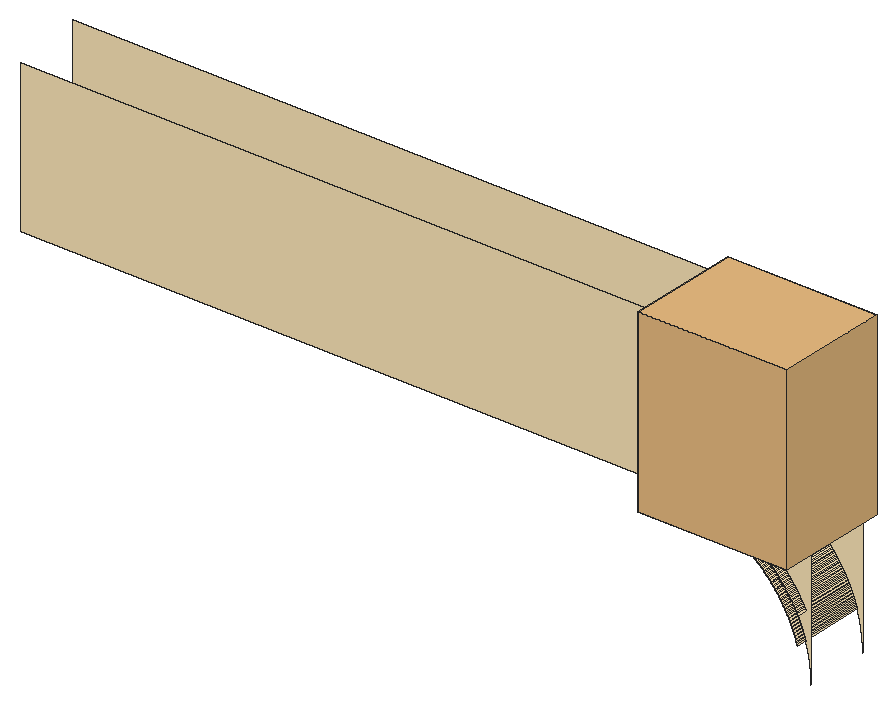
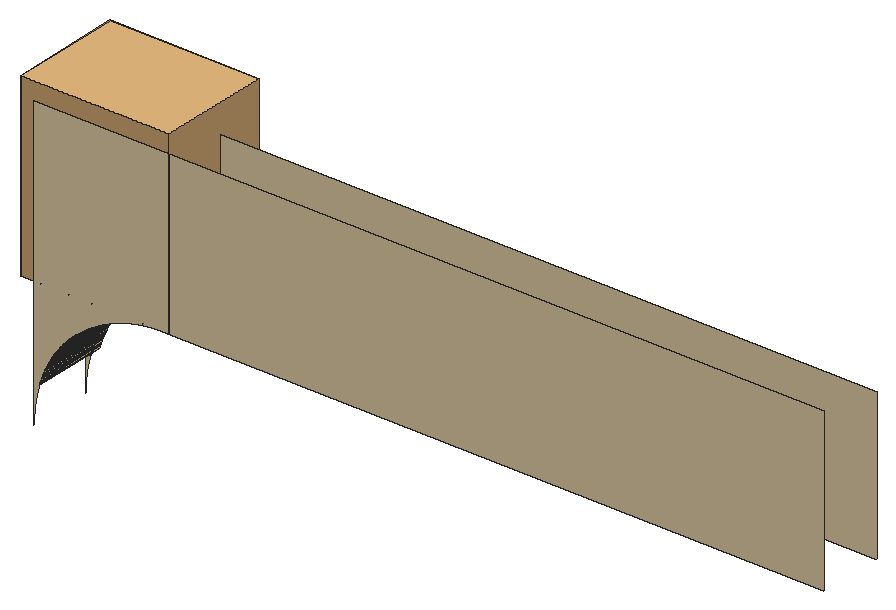
# SketchUp Ruby script. Lengths in inches.
U = 1.inch
M = Sketchup.active_model
def pt(a) = Geom::Point3d.new(a.map { |v| v * U })
def face(e, loops, mat)
  f = e.add_face(loops[0].map { |a| pt(a) })
  loops[1..].each { |l| e.add_face(l.map { |a| pt(a) }).erase! }
  f.material = f.back_material = mat if mat
  f
end
# faces: each face lists its corners as indices into pts; further lists are holes
def faces(e, pts, list, mat = nil) = list.each { |f| face(e, (f[0].is_a?(Array) ? f : [f]).map { |l| l.map { |i| pts[i] } }, mat) }
# xy, xz, yz: faces in a plane at the given z, y or x. An outline is a flat list of corners, or four numbers for a rectangle; further outlines are holes
def ring(l) = l.size == 4 ? [[l[0], l[1]], [l[2], l[1]], [l[2], l[3]], [l[0], l[3]]] : l.each_slice(2).to_a
def flat(e, list, mat, &to3) = list.each { |f| face(e, (f[0].is_a?(Array) ? f : [f]).map { |l| ring(l).map { |u, v| to3.(u, v) } }, mat) }
def xy(e, z, list, mat = nil) = flat(e, list, mat) { |x, y| [x, y, z] }
def xz(e, y, list, mat = nil) = flat(e, list, mat) { |x, z| [x, y, z] }
def yz(e, x, list, mat = nil) = flat(e, list, mat) { |y, z| [x, y, z] }
def lines(e, pts, list) = list.each { |a, b| e.add_line(pt(pts[a]), pt(pts[b])) }
# prism: a flat outline (further loops are holes) pulled along v
def prism(e, loops, v, mat = nil)
  f = face(e, loops, mat); d = Geom::Vector3d.new(v.map { |x| x * U })
  f.pushpull(f.normal.samedirection?(d) ? d.length : -d.length)
end
def box(e, o, s, mat = nil) = prism(e, [[o, [o[0] + s[0], o[1], o[2]], [o[0] + s[0], o[1] + s[1], o[2]], [o[0], o[1] + s[1], o[2]]]], [0, 0, s[2]], mat)
def at(x, y, z, deg = 0) = Geom::Transformation.translation(pt([x, y, z])) * Geom::Transformation.rotation(ORIGIN, Z_AXIS, deg.degrees)
def axes(o, x, y, z) = Geom::Transformation.new([*x, 0, *y, 0, *z, 0, *pt(o).to_a, 1])
def part(name) = M.definitions.add(name)
# library, detail: a bought-in or finely detailed component or shape, given as its bounding box
def library(name, o, s) = part(name).tap { |d| box(d.entities, o, s) }
def detail(e, o, s) = box(e.add_group.entities, o, s)
def put(e, d, t, mat = nil) = e.add_instance(d, t).tap { |i| i.material = mat if mat }
def group(e, t, mat = nil) = e.add_group.tap { |g| g.transformation = t; g.material = mat if mat }.entities
root = M.entities
M.materials.add("1026 AP 7946 SUNNY SIDE UP").color = [254, 231, 186]
c1 = library("climbing plant",[8874.76,-5589.78,-33.625],[50.13,38.07,87.16])
xz(root,227,[[177,222,176.999,222.236,176.995,222.471,176.99,222.707,176.981,222.942,176.971,223.178,176.958,223.413,176.943,223.648,176.926,223.883,176.906,224.118,176.884,224.352,176.86,224.587,176.834,224.821,176.805,225.055,176.774,225.288,176.74,225.522,176.705,225.754,176.667,225.987,176.626,226.219,176.584,226.451,176.539,226.682,176.492,226.913,176.442,227.143,176.391,227.373,176.337,227.603,176.281,227.832,176.222,228.06,176.162,228.287,176.099,228.515,176.034,228.741,175.967,228.967,175.897,229.192,175.825,229.416,175.751,229.64,175.675,229.863,175.597,230.085,175.517,230.307,175.434,230.527,175.349,230.747,175.262,230.966,175.173,231.184,175.082,231.402,174.989,231.618,174.893,231.833,174.795,232.048,174.696,232.261,174.594,232.474,174.49,232.685,174.384,232.896,174.276,233.105,174.166,233.314,174.054,233.521,173.94,233.727,173.824,233.932,173.706,234.136,173.585,234.338,173.463,234.54,173.339,234.74,173.213,234.939,173.085,235.137,172.955,235.334,172.823,235.529,172.69,235.723,172.554,235.916,172.416,236.107,172.277,236.297,172.136,236.485,171.993,236.673,171.848,236.858,171.701,237.043,171.552,237.225,171.402,237.407,171.25,237.587,171.096,237.765,170.94,237.942,170.783,238.117,170.624,238.291,170.463,238.463,170.3,238.634,170.136,238.803,169.971,238.971,169.803,239.136,169.634,239.3,169.463,239.463,169.291,239.624,169.117,239.783,168.942,239.94,168.765,240.096,168.587,240.25,168.407,240.402,168.225,240.552,168.043,240.701,167.858,240.848,167.673,240.993,167.485,241.136,167.297,241.277,167.107,241.416,166.916,241.554,166.723,241.69,166.529,241.823,166.334,241.955,166.137,242.085,165.939,242.213,165.74,242.339,165.54,242.463,165.338,242.585,165.136,242.706,164.932,242.824,164.727,242.94,164.521,243.054,164.314,243.166,164.105,243.276,163.896,243.384,163.685,243.49,163.474,243.594,163.261,243.696,163.048,243.795,162.833,243.893,162.618,243.989,162.402,244.082,162.184,244.173,161.966,244.262,161.747,244.349,161.527,244.434,161.307,244.517,161.085,244.597,160.863,244.675,160.64,244.751,160.416,244.825,160.192,244.897,159.967,244.967,159.741,245.034,159.515,245.099,159.287,245.162,159.06,245.222,158.832,245.281,158.603,245.337,158.373,245.391,158.143,245.442,157.913,245.492,157.682,245.539,157.451,245.584,157.219,245.626,156.987,245.667,156.754,245.705,156.522,245.74,156.288,245.774,156.055,245.805,155.821,245.834,155.587,245.86,155.352,245.884,155.118,245.906,154.883,245.926,154.648,245.943,154.413,245.958,154.178,245.971,153.942,245.981,153.707,245.99,153.471,245.995,153.236,245.999,153,246,30,246,30,276,177,276]],"1026 AP 7946 SUNNY SIDE UP")
p = [[177,215,222],[177,215,274],[29.764,215.001,274],[29.764,215.001,246],[30,215.001,246],[153,215,246],
  [153.002,215,246],[153.231,215,245.999],[153.236,215,245.999],[153.471,215,245.995],[153.707,215,245.99],[153.942,215,245.981],
  [154.178,215,245.971],[154.413,215,245.958],[154.648,215,245.943],[154.883,215,245.926],[155.118,215,245.906],[155.352,215,245.884],
  [155.587,215,245.86],[155.821,215,245.834],[156.055,215,245.805],[156.288,215,245.774],[156.522,215,245.74],[156.754,215,245.705],
  [156.987,215,245.667],[157.219,215,245.626],[157.451,215,245.584],[157.682,215,245.539],[157.913,215,245.492],[158.143,215,245.442],
  [158.373,215,245.391],[158.603,215,245.337],[158.832,215,245.281],[159.06,215,245.222],[159.287,215,245.162],[159.515,215,245.099],
  [159.741,215,245.034],[159.967,215,244.967],[160.192,215,244.897],[160.416,215,244.825],[160.64,215,244.751],[160.863,215,244.675],
  [161.085,215,244.597],[161.307,215,244.517],[161.527,215,244.434],[161.747,215,244.349],[161.966,215,244.262],[162.184,215,244.173],
  [162.402,215,244.082],[162.618,215,243.989],[162.833,215,243.893],[163.048,215,243.795],[163.261,215,243.696],[163.474,215,243.594],
  [163.685,215,243.49],[163.896,215,243.384],[164.105,215,243.276],[164.314,215,243.166],[164.521,215,243.054],[164.727,215,242.94],
  [164.932,215,242.824],[165.136,215,242.706],[165.338,215,242.585],[165.54,215,242.463],[165.74,215,242.339],[165.939,215,242.213],
  [166.137,215,242.085],[166.334,215,241.955],[166.529,215,241.823],[166.723,215,241.69],[166.916,215,241.554],[167.107,215,241.416],
  [167.297,215,241.277],[167.485,215,241.136],[167.673,215,240.993],[167.858,215,240.848],[168.043,215,240.701],[168.225,215,240.552],
  [168.407,215,240.402],[168.587,215,240.25],[168.765,215,240.096],[168.942,215,239.94],[169.117,215,239.783],[169.291,215,239.624],
  [169.463,215,239.463],[169.634,215,239.3],[169.803,215,239.136],[169.971,215,238.971],[170.136,215,238.803],[170.3,215,238.634],
  [170.463,215,238.463],[170.624,215,238.291],[170.783,215,238.117],[170.94,215,237.942],[171.096,215,237.765],[171.25,215,237.587],
  [171.402,215,237.407],[171.552,215,237.225],[171.701,215,237.043],[171.848,215,236.858],[171.993,215,236.673],[172.136,215,236.485],
  [172.277,215,236.297],[172.416,215,236.107],[172.554,215,235.916],[172.69,215,235.723],[172.823,215,235.529],[172.955,215,235.334],
  [173.085,215,235.137],[173.213,215,234.939],[173.339,215,234.74],[173.463,215,234.54],[173.585,215,234.338],[173.706,215,234.136],
  [173.824,215,233.932],[173.94,215,233.727],[174.054,215,233.521],[174.166,215,233.314],[174.276,215,233.105],[174.384,215,232.896],
  [174.49,215,232.685],[174.594,215,232.474],[174.696,215,232.261],[174.795,215,232.048],[174.893,215,231.833],[174.989,215,231.618],
  [175.082,215,231.402],[175.173,215,231.184],[175.262,215,230.966],[175.349,215,230.747],[175.434,215,230.527],[175.517,215,230.307],
  [175.597,215,230.085],[175.675,215,229.863],[175.751,215,229.64],[175.825,215,229.416],[175.897,215,229.192],[175.967,215,228.967],
  [176.034,215,228.741],[176.099,215,228.515],[176.162,215,228.287],[176.222,215,228.06],[176.281,215,227.832],[176.337,215,227.603],
  [176.391,215,227.373],[176.442,215,227.143],[176.492,215,226.913],[176.539,215,226.682],[176.584,215,226.451],[176.626,215,226.219],
  [176.667,215,225.987],[176.705,215,225.754],[176.74,215,225.522],[176.774,215,225.288],[176.805,215,225.055],[176.834,215,224.821],
  [176.86,215,224.587],[176.884,215,224.352],[176.906,215,224.118],[176.926,215,223.883],[176.943,215,223.648],[176.958,215,223.413],
  [176.971,215,223.178],[176.981,215,222.942],[176.99,215,222.707],[176.995,215,222.471],[176.999,215,222.236],[175.967,215.099,228.967],
  [176.034,215.099,228.741],[175.897,213.099,229.192],[175.967,213.099,228.967],[175.897,215.099,229.192],[175.967,227,228.967],[175.897,227,229.192],
  [175.825,213.099,229.416],[175.825,215.099,229.416],[175.825,227,229.416],[175.751,213.099,229.64],[175.751,215.099,229.64],[175.751,227,229.64],
  [175.675,213.099,229.863],[175.675,215.099,229.863],[175.675,227,229.863],[175.597,213.099,230.085],[175.597,215.099,230.085],[175.597,227,230.085],
  [175.517,213.099,230.307],[175.517,215.099,230.307],[175.517,227,230.307],[175.434,213.099,230.527],[175.434,215.099,230.527],[175.434,227,230.527],
  [175.349,213.099,230.747],[175.349,215.099,230.747],[175.349,227,230.747],[175.262,213.099,230.966],[175.262,215.099,230.966],[175.262,227,230.966],
  [175.173,213.099,231.184],[175.173,215.099,231.184],[175.173,227,231.184],[175.082,213.099,231.402],[175.082,215.099,231.402],[175.082,227,231.402],
  [174.989,213.099,231.618],[174.989,215.099,231.618],[174.989,227,231.618],[174.893,213.099,231.833],[174.893,215.099,231.833],[174.893,227,231.833],
  [174.795,213.099,232.048],[174.795,215.099,232.048],[174.795,227,232.048],[174.696,213.099,232.261],[174.696,215.099,232.261],[174.696,227,232.261],
  [174.594,213.099,232.474],[174.594,215.099,232.474],[174.594,227,232.474],[174.49,213.099,232.685],[174.49,215.099,232.685],[174.49,227,232.685],
  [174.384,213.099,232.896],[174.384,215.099,232.896],[174.384,227,232.896],[174.276,213.099,233.105],[174.276,215.099,233.105],[174.276,227,233.105],
  [174.166,213.099,233.314],[174.166,215.099,233.314],[174.166,227,233.314],[174.054,213.099,233.521],[174.054,215.099,233.521],[174.054,227,233.521],
  [173.94,213.099,233.727],[173.94,215.099,233.727],[173.94,227,233.727],[173.824,213.099,233.932],[173.824,215.099,233.932],[173.824,227,233.932],
  [173.706,213.099,234.136],[173.706,215.099,234.136],[173.706,227,234.136],[176.049,213.099,234.031],[176.049,215.099,234.031],[175.93,215.099,234.256],
  [175.93,213.099,234.256],[173.585,213.099,234.338],[173.585,215.099,234.338],[173.585,227,234.338],[173.463,213.099,234.54],[175.809,215.099,234.481],
  [175.809,213.099,234.481],[173.463,215.099,234.54],[173.463,227,234.54],[173.339,213.099,234.74],[175.685,215.099,234.704],[175.685,213.099,234.704],
  [173.339,215.099,234.74],[173.339,227,234.74],[173.213,213.099,234.939],[175.559,215.099,234.926],[175.559,213.099,234.926],[173.213,215.099,234.939],
  [173.213,227,234.939],[173.085,213.099,235.137],[175.431,215.099,235.147],[175.431,213.099,235.147],[173.085,215.099,235.137],[173.085,227,235.137],
  [172.955,213.099,235.334],[175.301,215.099,235.367],[175.301,213.099,235.367],[172.955,215.099,235.334],[172.955,227,235.334],[172.823,213.099,235.529],
  [172.823,215.099,235.529],[172.823,227,235.529],[175.169,215.099,235.585],[175.169,213.099,235.585],[172.69,213.099,235.723],[172.69,215.099,235.723],
  [172.69,227,235.723],[175.034,215.099,235.802],[175.034,213.099,235.802],[172.554,213.099,235.916],[172.554,215.099,235.916],[172.554,227,235.916],
  [174.898,215.099,236.018],[174.898,213.099,236.018],[172.416,213.099,236.107],[172.416,215.099,236.107],[172.416,227,236.107],[174.759,215.099,236.232],
  [174.759,213.099,236.232],[172.277,213.099,236.297],[172.277,215.099,236.297],[172.277,227,236.297],[174.618,215.099,236.445],[174.618,213.099,236.445],
  [172.136,213.099,236.485],[172.136,215.099,236.485],[172.136,227,236.485],[174.475,215.099,236.656],[174.475,213.099,236.656],[171.993,213.099,236.673],
  [171.993,215.099,236.673],[171.993,227,236.673],[171.848,213.099,236.858],[174.33,215.099,236.867],[174.33,213.099,236.867],[171.848,215.099,236.858],
  [171.848,227,236.858],[171.701,213.099,237.043],[174.183,215.099,237.075],[174.183,213.099,237.075],[171.701,215.099,237.043],[171.701,227,237.043],
  [171.552,213.099,237.225],[171.552,215.099,237.225],[171.552,227,237.225],[174.034,215.099,237.282],[174.034,213.099,237.282],[171.402,213.099,237.407],
  [171.402,215.099,237.407],[171.402,227,237.407],[173.883,215.099,237.488],[173.883,213.099,237.488],[171.25,213.099,237.587],[171.25,215.099,237.587],
  [171.25,227,237.587],[173.73,215.099,237.692],[173.73,213.099,237.692],[171.096,213.099,237.765],[171.096,215.099,237.765],[171.096,227,237.765],
  [173.575,215.099,237.895],[173.575,213.099,237.895],[170.94,213.099,237.942],[170.94,215.099,237.942],[170.94,227,237.942],[170.783,213.099,238.117],
  [173.418,215.099,238.096],[173.418,213.099,238.096],[170.783,215.099,238.117],[170.783,227,238.117],[170.624,213.099,238.291],[173.259,215.099,238.296],
  [173.259,213.099,238.296],[170.624,215.099,238.291],[170.624,227,238.291],[170.463,213.099,238.463],[173.098,215.099,238.494],[173.098,213.099,238.494],
  [170.463,215.099,238.463],[170.463,227,238.463],[170.3,213.099,238.634],[172.935,215.099,238.691],[172.935,213.099,238.691],[170.3,215.099,238.634],
  [170.3,227,238.634],[170.136,213.099,238.803],[170.136,215.099,238.803],[170.136,227,238.803],[172.771,215.099,238.886],[172.771,213.099,238.886],
  [169.971,213.099,238.971],[169.971,215.099,238.971],[169.971,227,238.971],[172.604,215.099,239.079],[172.604,213.099,239.079],[169.803,213.099,239.136],
  [169.803,215.099,239.136],[169.803,227,239.136],[169.634,213.099,239.3],[172.435,215.099,239.271],[172.435,213.099,239.271],[169.634,215.099,239.3],
  [169.634,227,239.3],[169.463,213.099,239.463],[172.265,215.099,239.461],[172.265,213.099,239.461],[169.463,215.099,239.463],[169.463,227,239.463],
  [169.291,213.099,239.624],[172.092,215.099,239.649],[172.092,213.099,239.649],[169.291,215.099,239.624],[169.291,227,239.624],[169.117,213.099,239.783],
  [171.918,215.099,239.835],[171.918,213.099,239.835],[169.117,215.099,239.783],[169.117,227,239.783],[168.942,213.099,239.94],[171.742,215.099,240.02],
  [171.742,213.099,240.02],[168.942,215.099,239.94],[168.942,227,239.94],[168.765,213.099,240.096],[168.765,215.099,240.096],[168.765,227,240.096],
  [171.564,215.099,240.203],[171.564,213.099,240.203],[168.587,213.099,240.25],[168.587,215.099,240.25],[168.587,227,240.25],[168.407,213.099,240.402],
  [171.385,215.099,240.385],[171.385,213.099,240.385],[168.407,215.099,240.402],[168.407,227,240.402],[168.225,213.099,240.552],[171.203,215.099,240.564],
  [171.203,213.099,240.564],[168.225,215.099,240.552],[168.225,227,240.552],[168.043,213.099,240.701],[171.02,215.099,240.742],[171.02,213.099,240.742],
  [168.043,215.099,240.701],[168.043,227,240.701],[167.858,213.099,240.848],[170.835,215.099,240.918],[170.835,213.099,240.918],[167.858,215.099,240.848],
  [167.858,227,240.848],[167.673,213.099,240.993],[167.673,215.099,240.993],[167.673,227,240.993],[170.649,215.099,241.092],[170.649,213.099,241.092],
  [167.485,213.099,241.136],[167.485,215.099,241.136],[167.485,227,241.136],[167.297,213.099,241.277],[170.461,215.099,241.265],[170.461,213.099,241.265],
  [167.297,215.099,241.277],[167.297,227,241.277],[167.107,213.099,241.416],[170.271,215.099,241.435],[170.271,213.099,241.435],[167.107,215.099,241.416],
  [167.107,227,241.416],[166.916,213.099,241.554],[170.079,215.099,241.604],[170.079,213.099,241.604],[166.916,215.099,241.554],[166.916,227,241.554],
  [166.723,213.099,241.69],[169.886,215.099,241.771],[169.886,213.099,241.771],[166.723,215.099,241.69],[166.723,227,241.69],[166.529,213.099,241.823],
  [166.529,215.099,241.823],[166.529,227,241.823],[166.334,213.099,241.955],[169.691,215.099,241.935],[169.691,213.099,241.935],[166.334,215.099,241.955],
  [166.334,227,241.955],[169.494,215.099,242.098],[169.494,213.099,242.098],[166.137,213.099,242.085],[166.137,215.099,242.085],[166.137,227,242.085],
  [165.939,213.099,242.213],[169.296,215.099,242.259],[169.296,213.099,242.259],[165.939,215.099,242.213],[165.939,227,242.213],[165.74,213.099,242.339],
  [165.74,215.099,242.339],[165.74,227,242.339],[165.54,213.099,242.463],[169.096,215.099,242.418],[169.096,213.099,242.418],[165.54,215.099,242.463],
  [165.54,227,242.463],[168.895,215.099,242.575],[168.895,213.099,242.575],[165.338,213.099,242.585],[165.338,215.099,242.585],[165.338,227,242.585],
  [168.692,215.099,242.73],[168.692,213.099,242.73],[168.488,215.099,242.883],[168.488,213.099,242.883],[168.282,215.099,243.034],[168.282,213.099,243.034],
  [168.075,215.099,243.183],[168.075,213.099,243.183],[167.867,215.099,243.33],[167.867,213.099,243.33],[167.656,215.099,243.475],[167.656,213.099,243.475],
  [167.445,215.099,243.618],[167.445,213.099,243.618],[167.232,215.099,243.759],[167.232,213.099,243.759],[167.018,215.099,243.898],[167.018,213.099,243.898],
  [166.802,215.099,244.034],[166.802,213.099,244.034],[166.585,215.099,244.169],[166.585,213.099,244.169],[166.367,215.099,244.301],[166.367,213.099,244.301],
  [166.147,215.099,244.431],[166.147,213.099,244.431],[165.926,215.099,244.559],[165.926,213.099,244.559],[165.704,215.099,244.685],[165.704,213.099,244.685],
  [165.481,215.099,244.809],[165.481,213.099,244.809]]
faces(root,p,[[0,1,2,3,4,5,6,7,8,9,10,11,12,13,14,15,16,17,18,19,20,21,22,23,24,25,26,27,28,29,30,31,32,33,34,35,36,37,38,39,40,41,42,43,44,45,46,47,48,49,50,51,52,53,54,55,56,57,58,59,60,61,62,63,64,65,66,67,68,69,70,71,72,73,74,75,76,77,78,79,80,81,82,83,84,85,86,87,88,89,90,91,92,93,94,95,96,97,98,99,100,101,102,103,104,105,106,107,108,109,110,111,112,113,114,115,116,117,118,119,120,121,122,123,124,125,126,127,128,129,130,131,132,133,134,135,136,137,138,139,140,141,142,143,144,145,146,147,148,149,150,151,152,153,154,155,156,157,158,159,160,161,162,163,164,165,166],[137,167,168,138],[169,136,137,170],[136,171,167,137],[172,167,171,173],[174,135,136,169],[135,175,171,136],[173,171,175,176],
  [177,134,135,174],[134,178,175,135],[176,175,178,179],[180,133,134,177],[133,181,178,134],[179,178,181,182],[183,132,133,180],[132,184,181,133],
  [182,181,184,185],[186,131,132,183],[131,187,184,132],[185,184,187,188],[189,130,131,186],[130,190,187,131],[188,187,190,191],[192,129,130,189],
  [129,193,190,130],[191,190,193,194],[195,128,129,192],[128,196,193,129],[194,193,196,197],[198,127,128,195],[127,199,196,128],[197,196,199,200],
  [201,126,127,198],[126,202,199,127],[200,199,202,203],[204,125,126,201],[125,205,202,126],[203,202,205,206],[207,124,125,204],[124,208,205,125],
  [206,205,208,209],[210,123,124,207],[123,211,208,124],[209,208,211,212],[213,122,123,210],[122,214,211,123],[212,211,214,215],[216,121,122,213],
  [121,217,214,122],[215,214,217,218],[219,120,121,216],[120,220,217,121],[218,217,220,221],[222,119,120,219],[119,223,220,120],[221,220,223,224],
  [225,118,119,222],[118,226,223,119],[224,223,226,227],[228,117,118,225],[117,229,226,118],[227,226,229,230],[231,116,117,228],[116,232,229,117],
  [230,229,232,233],[234,115,116,231],[115,235,232,116],[233,232,235,236],[237,114,115,234],[114,238,235,115],[236,235,238,239],[240,113,114,237],
  [113,241,238,114],[239,238,241,242],[243,244,245,246],[247,112,113,240],[112,248,241,113],[242,241,248,249],[250,111,112,247],[246,245,251,252],
  [111,253,248,112],[249,248,253,254],[255,110,111,250],[252,251,256,257],[110,258,253,111],[254,253,258,259],[260,109,110,255],[257,256,261,262],
  [109,263,258,110],[259,258,263,264],[265,108,109,260],[262,261,266,267],[108,268,263,109],[264,263,268,269],[270,107,108,265],[267,266,271,272],
  [107,273,268,108],[269,268,273,274],[275,106,107,270],[106,276,273,107],[274,273,276,277],[272,271,278,279],[280,105,106,275],[105,281,276,106],
  [277,276,281,282],[279,278,283,284],[285,104,105,280],[104,286,281,105],[282,281,286,287],[284,283,288,289],[290,103,104,285],[103,291,286,104],
  [287,286,291,292],[289,288,293,294],[295,102,103,290],[102,296,291,103],[292,291,296,297],[294,293,298,299],[300,101,102,295],[101,301,296,102],
  [297,296,301,302],[299,298,303,304],[305,100,101,300],[100,306,301,101],[302,301,306,307],[308,99,100,305],[304,303,309,310],[99,311,306,100],
  [307,306,311,312],[313,98,99,308],[310,309,314,315],[98,316,311,99],[312,311,316,317],[318,97,98,313],[97,319,316,98],[317,316,319,320],
  [315,314,321,322],[323,96,97,318],[96,324,319,97],[320,319,324,325],[322,321,326,327],[328,95,96,323],[95,329,324,96],[325,324,329,330],
  [327,326,331,332],[333,94,95,328],[94,334,329,95],[330,329,334,335],[332,331,336,337],[338,93,94,333],[93,339,334,94],[335,334,339,340],
  [341,92,93,338],[337,336,342,343],[92,344,339,93],[340,339,344,345],[346,91,92,341],[343,342,347,348],[91,349,344,92],[345,344,349,350],
  [351,90,91,346],[348,347,352,353],[90,354,349,91],[350,349,354,355],[356,89,90,351],[353,352,357,358],[89,359,354,90],[355,354,359,360],
  [361,88,89,356],[88,362,359,89],[360,359,362,363],[358,357,364,365],[366,87,88,361],[87,367,362,88],[363,362,367,368],[365,364,369,370],
  [371,86,87,366],[86,372,367,87],[368,367,372,373],[374,85,86,371],[370,369,375,376],[85,377,372,86],[373,372,377,378],[379,84,85,374],
  [376,375,380,381],[84,382,377,85],[378,377,382,383],[384,83,84,379],[381,380,385,386],[83,387,382,84],[383,382,387,388],[389,82,83,384],
  [386,385,390,391],[82,392,387,83],[388,387,392,393],[394,81,82,389],[391,390,395,396],[81,397,392,82],[393,392,397,398],[399,80,81,394],
  [80,400,397,81],[398,397,400,401],[396,395,402,403],[404,79,80,399],[79,405,400,80],[401,400,405,406],[407,78,79,404],[403,402,408,409],
  [78,410,405,79],[406,405,410,411],[412,77,78,407],[409,408,413,414],[77,415,410,78],[411,410,415,416],[417,76,77,412],[414,413,418,419],
  [76,420,415,77],[416,415,420,421],[422,75,76,417],[419,418,423,424],[75,425,420,76],[421,420,425,426],[427,74,75,422],[74,428,425,75],
  [426,425,428,429],[424,423,430,431],[432,73,74,427],[73,433,428,74],[429,428,433,434],[435,72,73,432],[431,430,436,437],[72,438,433,73],
  [434,433,438,439],[440,71,72,435],[437,436,441,442],[71,443,438,72],[439,438,443,444],[445,70,71,440],[442,441,446,447],[70,448,443,71],
  [444,443,448,449],[450,69,70,445],[447,446,451,452],[69,453,448,70],[449,448,453,454],[455,68,69,450],[68,456,453,69],[454,453,456,457],
  [458,67,68,455],[452,451,459,460],[67,461,456,68],[457,456,461,462],[460,459,463,464],[465,66,67,458],[66,466,461,67],[462,461,466,467],
  [468,65,66,465],[464,463,469,470],[65,471,466,66],[467,466,471,472],[473,64,65,468],[64,474,471,65],[472,471,474,475],[476,63,64,473],
  [470,469,477,478],[63,479,474,64],[475,474,479,480],[478,477,481,482],[483,62,63,476],[62,484,479,63],[480,479,484,485],[482,481,486,487],
  [487,486,488,489],[489,488,490,491],[491,490,492,493],[493,492,494,495],[495,494,496,497],[497,496,498,499],[499,498,500,501],[501,500,502,503],
  [503,502,504,505],[505,504,506,507],[507,506,508,509],[509,508,510,511],[511,510,512,513],[513,512,514,515],[515,514,516,517]],"1026 AP 7946 SUNNY SIDE UP")
put(root,c1,axes([-4729.15,3280.44,258.875],[0.55,0,0],[0,0.55,0],[0,0,0.3829]),"1026 AP 7946 SUNNY SIDE UP")
